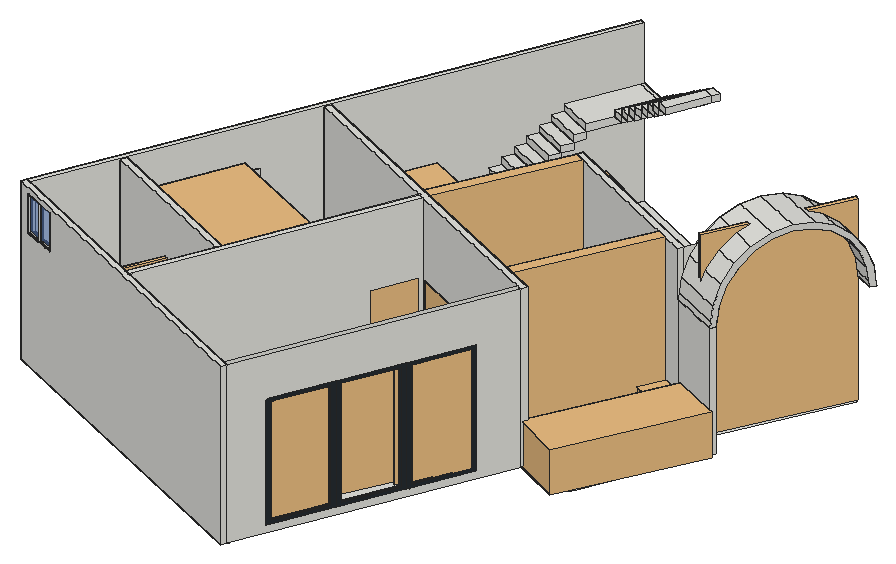
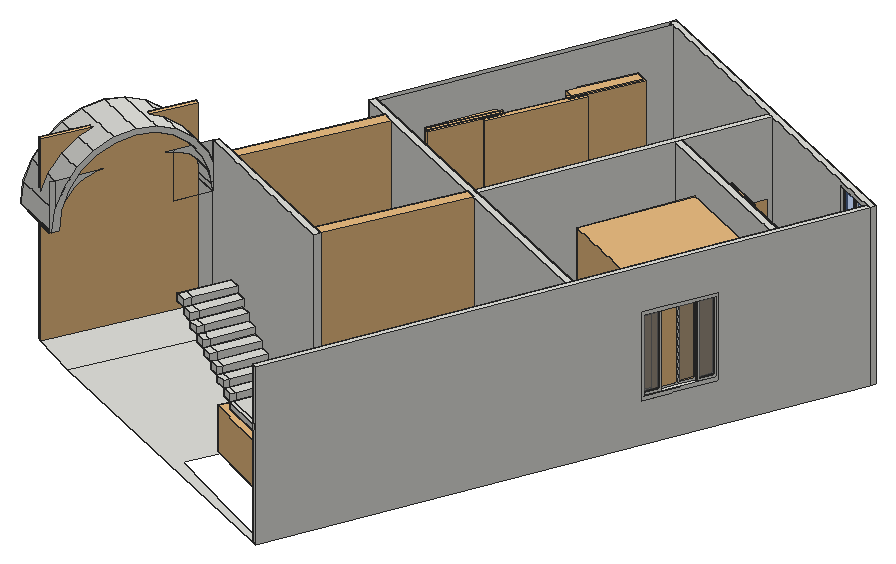
# SketchUp Ruby script. Lengths in inches.
U = 1.inch
M = Sketchup.active_model
def pt(a) = Geom::Point3d.new(a.map { |v| v * U })
def face(e, loops, mat)
  f = e.add_face(loops[0].map { |a| pt(a) })
  loops[1..].each { |l| e.add_face(l.map { |a| pt(a) }).erase! }
  f.material = f.back_material = mat if mat
  f
end
# faces: each face lists its corners as indices into pts; further lists are holes
def faces(e, pts, list, mat = nil) = list.each { |f| face(e, (f[0].is_a?(Array) ? f : [f]).map { |l| l.map { |i| pts[i] } }, mat) }
# xy, xz, yz: faces in a plane at the given z, y or x. An outline is a flat list of corners, or four numbers for a rectangle; further outlines are holes
def ring(l) = l.size == 4 ? [[l[0], l[1]], [l[2], l[1]], [l[2], l[3]], [l[0], l[3]]] : l.each_slice(2).to_a
def flat(e, list, mat, &to3) = list.each { |f| face(e, (f[0].is_a?(Array) ? f : [f]).map { |l| ring(l).map { |u, v| to3.(u, v) } }, mat) }
def xy(e, z, list, mat = nil) = flat(e, list, mat) { |x, y| [x, y, z] }
def xz(e, y, list, mat = nil) = flat(e, list, mat) { |x, z| [x, y, z] }
def yz(e, x, list, mat = nil) = flat(e, list, mat) { |y, z| [x, y, z] }
def lines(e, pts, list) = list.each { |a, b| e.add_line(pt(pts[a]), pt(pts[b])) }
# prism: a flat outline (further loops are holes) pulled along v
def prism(e, loops, v, mat = nil)
  f = face(e, loops, mat); d = Geom::Vector3d.new(v.map { |x| x * U })
  f.pushpull(f.normal.samedirection?(d) ? d.length : -d.length)
end
def box(e, o, s, mat = nil) = prism(e, [[o, [o[0] + s[0], o[1], o[2]], [o[0] + s[0], o[1] + s[1], o[2]], [o[0], o[1] + s[1], o[2]]]], [0, 0, s[2]], mat)
def at(x, y, z, deg = 0) = Geom::Transformation.translation(pt([x, y, z])) * Geom::Transformation.rotation(ORIGIN, Z_AXIS, deg.degrees)
def axes(o, x, y, z) = Geom::Transformation.new([*x, 0, *y, 0, *z, 0, *pt(o).to_a, 1])
def part(name) = M.definitions.add(name)
# library, detail: a bought-in or finely detailed component or shape, given as its bounding box
def library(name, o, s) = part(name).tap { |d| box(d.entities, o, s) }
def detail(e, o, s) = box(e.add_group.entities, o, s)
def put(e, d, t, mat = nil) = e.add_instance(d, t).tap { |i| i.material = mat if mat }
def group(e, t, mat = nil) = e.add_group.tap { |g| g.transformation = t; g.material = mat if mat }.entities
root = M.entities
M.materials.add("Wine2").color = [0, 0, 0]
M.materials["Wine2"].alpha = 0
M.materials.add("[0130_Gainsboro]").color = [39, 45, 50]
M.materials.add("[Translucent Glass Blue]").color = [100, 149, 237]
M.materials["[Translucent Glass Blue]"].alpha = 0.5
M.materials.add("[Translucent_Glass_Gray]4").color = [128, 128, 128]
M.materials["[Translucent_Glass_Gray]4"].alpha = 0.5
c1 = library("KOŁO+DRZWI+WNĘKOWE+SKRZYDŁOWE+NEXT+80,+PRAWOSTRONNE+HDRF80R\#",[0.43,0.44,0],[31.07,2.7,98.875])
c2 = library("porta 4",[0.2,-5.42,1.33],[46.55,4.72,83.21])
c3 = library("KOŁO+DRZWI+WNĘKOWE+SKRZYDŁOWE+NEXT+80,+PRAWOSTRONNE+HDRF80R",[-3.72,0,0],[35.22,3.14,98.875])
c4 = library("Group\#121",[0,0,0],[95.11,121,36.98])
c5 = library("Group\#46",[0,0,0],[59.88,84.57,74.8])
c6 = part("Group\#12")
box(c6.entities,[0,0,0],[5,144,144])
c7 = library("Bedroom furniture set",[0,-4.61,0],[113.04,95.21,114.59])
c8 = library("Group\#66",[0,0,0],[120.1,9.95,144])
c9 = library("Group\#8",[0,0,0],[126.47,47.76,36.98])
c10 = part("Group\#4")
prism(c10.entities,[[[0,298,0],[0,-5,0],[0,-5,144],[0,298,144]],[[0,39.33,108],[0,39.33,139.52],[0,7,139.52],[0,7,108]]],[5,0,0])
c11 = part("Group\#11")
prism(c11.entities,[[[0,149,0],[0,41.99,0],[0,41.99,78],[0,2.99,78],[0,2.99,0],[0,-149,0],[0,-149,144],[0,149,144]]],[5,0,0])
c12 = library("Kohler_Balast_1935.skp\#1",[-38.83,-18.45,0],[74.81,42.21,2.86])
c13 = library("window 1",[0,0,0],[3.9375,118.11,177.17])
c14 = part("Group\#74")
xy(c14.entities,0,[[0,-0.98,43.07,0],[0,0,43.07,1.4]],"[0130_Gainsboro]")
xy(c14.entities,0.3,[[0.3,-1.43,42.77,-0.98]],"[0130_Gainsboro]")
xy(c14.entities,2.95,[[2.95,-1.43,40.12,-0.63],[2.95,-0.63,40.12,0],[2.95,0,40.12,0.64],[2.95,0.64,40.12,1.4]],"[0130_Gainsboro]")
xy(c14.entities,3.54,[[3.54,-0.63,39.53,0],[3.54,0,39.53,0.64]],"[0130_Gainsboro]")
xy(c14.entities,111.8125,[[3.54,-0.63,39.53,0],[3.54,0,39.53,0.64]],"[0130_Gainsboro]")
xy(c14.entities,112.4,[[2.95,-1.43,40.12,-0.63],[2.95,-0.63,40.12,0],[2.95,0,40.12,0.64],[2.95,0.64,40.12,1.4]],"[0130_Gainsboro]")
xy(c14.entities,115.05,[[0.3,-1.43,42.77,-0.98]],"[0130_Gainsboro]")
xy(c14.entities,115.35,[[0,-0.98,43.07,0],[0,0,43.07,1.4]],"[0130_Gainsboro]")
xz(c14.entities,-1.43,[[[0.3,0.3,42.77,115.05],[2.95,2.95,40.12,112.4]]],"[0130_Gainsboro]")
xz(c14.entities,-0.98,[[[0,0,43.07,115.35],[0.3,0.3,42.77,115.05]]],"[0130_Gainsboro]")
xz(c14.entities,-0.63,[[[2.95,2.95,40.12,112.4],[3.54,3.54,39.53,111.8125]]],"[0130_Gainsboro]")
xz(c14.entities,0,[[3.54,3.54,39.53,111.8125]],"Wine2")
xz(c14.entities,0,[[[0,0,43.07,115.35],[2.95,2.95,40.12,112.4]],[[2.95,2.95,40.12,112.4],[3.54,3.54,39.53,111.8125]]],"[0130_Gainsboro]")
xz(c14.entities,0.64,[[[2.95,2.95,40.12,112.4],[3.54,3.54,39.53,111.8125]]],"[0130_Gainsboro]")
xz(c14.entities,1.4,[[[0,0,43.07,115.35],[2.95,2.95,40.12,112.4]]],"[0130_Gainsboro]")
yz(c14.entities,0,[[-0.98,0,0,115.35],[0,0,1.4,115.35]],"[0130_Gainsboro]")
yz(c14.entities,0.3,[[-1.43,0.3,-0.98,115.05]],"[0130_Gainsboro]")
yz(c14.entities,2.95,[[-1.43,2.95,-0.63,112.4],[-0.63,2.95,0,112.4],[0,2.95,0.64,112.4],[0.64,2.95,1.4,112.4]],"[0130_Gainsboro]")
yz(c14.entities,3.54,[[-0.63,3.54,0,111.8125],[0,3.54,0.64,111.8125]],"[0130_Gainsboro]")
yz(c14.entities,39.53,[[-0.63,3.54,0,111.8125],[0,3.54,0.64,111.8125]],"[0130_Gainsboro]")
yz(c14.entities,40.12,[[-1.43,2.95,-0.63,112.4],[-0.63,2.95,0,112.4],[0,2.95,0.64,112.4],[0.64,2.95,1.4,112.4]],"[0130_Gainsboro]")
yz(c14.entities,42.77,[[-1.43,0.3,-0.98,115.05]],"[0130_Gainsboro]")
yz(c14.entities,43.07,[[-0.98,0,0,115.35],[0,0,1.4,115.35]],"[0130_Gainsboro]")
c15 = part("Glazed door assembly")
put(c15.entities,c14,axes([90.57,1.43,0],[1.05148,0,0],[0,1,0],[0,0,1]))
put(c15.entities,c14,axes([0,1.43,0],[1.05148,0,0],[0,1,0],[0,0,1]))
put(c15.entities,c14,axes([45.29,1.43,0],[1.05148,0,0],[0,1,0],[0,0,1]))
c16 = library("Group8\#1",[-48.75,-20.06,-0.03],[97.5,40.12,31.8])
c17 = library("3d flower - flower pot",[-12.2,-15.73,0],[29.88,29.15,27.8])
c18 = library("Dining table set",[0,0,0],[65.45,109.33,43.4])
c19 = library("Group14",[-64.97,9.24,0.31],[138.52,9.93,292.57])
c20 = library("Group16",[86.37,-10.76,76.46],[21.79,14.87,35.97])
c21 = library("Group22",[48.82,-10.91,0.23],[97.72,18.57,293.12])
c22 = library("Group24",[44.03,2.01,0.26],[103.73,11,292.35])
c23 = library("Group27",[-106.21,-10.76,76.46],[21.8,14.87,35.97])
c24 = library("Group35",[-145.81,2.01,0.26],[103.73,11,292.35])
c25 = library("Group33",[-144.59,-10.91,0.23],[97.72,18.57,293.12])
c26 = part("Group\#71")
put(c26.entities,c19,at(145.81,10.91,-0.23))
put(c26.entities,c20,at(145.81,10.91,-0.23))
put(c26.entities,c21,at(145.81,10.91,-0.23))
put(c26.entities,c22,at(145.81,10.91,-0.23))
put(c26.entities,c23,at(145.81,10.91,-0.23))
put(c26.entities,c24,at(145.81,10.91,-0.23))
put(c26.entities,c25,at(145.81,10.91,-0.23))
c27 = library("Group13\#1",[-103.57,-19.82,-0.03],[42.43,40.67,31.4])
c28 = part("Group\#117")
xy(c28.entities,0,[[0,0,36,10]])
g1 = group(c28.entities,at(-0.41,0,0))
g2 = group(g1,at(0,0,0))
xy(g2,6,[[0.41,0,36.41,10]])
xz(g2,0,[[0.41,0,36.41,6]])
xz(g2,10,[[0.41,0,36.41,6]])
yz(g2,0.41,[[0,0,10,6]])
yz(g2,36.41,[[0,0,10,6]])
c29 = library("bathroom kit",[-10.19,-11.89,-0.14],[22.08,39.51,30.77])
c30 = library("Shower_03.skp",[-9.2,-8.46,-0.03],[13.92,58.47,24.25])
c31 = part("Component\#36")
prism(c31.entities,[[[0,70.87,0],[0,0,0],[0,0,47.24],[0,70.87,47.24]],[[0,1.97,1.97],[0,68.9,1.97],[0,68.9,45.28],[0,1.97,45.28]]],[7.875,0,0])
c32 = part("Component\#34")
xy(c32.entities,0,[[0,0,3.9375,16.73]])
xy(c32.entities,0.98,[[0,0.98,1.77,15.75],[1.77,0.98,2.85,15.75],[2.85,0.98,3.9375,15.75]])
xy(c32.entities,42.32,[[0,0.98,1.77,15.75],[1.77,0.98,2.85,15.75],[2.85,0.98,3.9375,15.75]])
xy(c32.entities,43.31,[[0,0,3.9375,16.73]])
xz(c32.entities,0,[[0,0,3.9375,43.31]])
xz(c32.entities,0.98,[[0,0.98,1.77,42.32],[1.77,0.98,2.85,42.32],[2.85,0.98,3.9375,42.32]])
xz(c32.entities,15.75,[[0,0.98,1.77,42.32],[1.77,0.98,2.85,42.32],[2.85,0.98,3.9375,42.32]])
xz(c32.entities,16.73,[[0,0,3.9375,43.31]])
yz(c32.entities,0,[[[0,0,16.73,43.31],[0.98,0.98,15.75,42.32]]])
yz(c32.entities,1.77,[[0.98,0.98,15.75,42.32]],"[Translucent_Glass_Gray]4")
yz(c32.entities,2.85,[[0.98,0.98,15.75,42.32]],"[Translucent_Glass_Gray]4")
yz(c32.entities,3.9375,[[[0,0,16.73,43.31],[0.98,0.98,15.75,42.32]]])
c33 = part("simple window")
p = [[0,68.9,1.97],[0,35.43,1.97]]
lines(c33.entities,p,[[0,1]])
put(c33.entities,c31,at(0,0,0))
put(c33.entities,c32,axes([1.14,52.17,1.97],[0.71,0,0],[0,1,0],[0,0,1]))
put(c33.entities,c32,axes([1.14,1.97,1.97],[0.71,0,0],[0,1,0],[0,0,1]))
put(c33.entities,c32,axes([3.9375,18.7,1.97],[0.71,0,0],[0,1,0],[0,0,1]))
put(c33.entities,c32,axes([3.9375,35.43,1.97],[0.71,0,0],[0,1,0],[0,0,1]))
c34 = part("Group\#67")
xy(c34.entities,0,[[0,0,36,10]])
g3 = group(c34.entities,at(-0.41,0,0))
g4 = group(g3,at(0,0,0))
xy(g4,6,[[0.41,0,36.41,35.24]])
xz(g4,0,[[0.41,0,36.41,6]])
xz(g4,35.24,[[0.41,0,36.41,6]])
yz(g4,0.41,[[0,0,35.24,6]])
yz(g4,36.41,[[0,0,35.24,6]])
c35 = part("Group\#53")
xy(c35.entities,0,[[0,0,36,10]])
g5 = group(c35.entities,at(-0.41,0,0))
g6 = group(g5,at(0,0,0))
xy(g6,6,[[0.41,0,36.41,10]])
xz(g6,0,[[0.41,0,36.41,6]])
xz(g6,10,[[0.41,0,36.41,6]])
yz(g6,0.41,[[0,0,10,6]])
yz(g6,36.41,[[0,0,10,6]])
c36 = part("Janela aluminio")
xy(c36.entities,0,[[0,0,47.24,1.57],[23.62,1.57,47.24,2.76],[0,2.76,25.98,3.9375],[0,3.9375,47.24,5.91]])
xy(c36.entities,43.31,[[0,0,47.24,1.57],[23.62,1.57,47.24,2.76],[0,2.76,0,5.91,47.24,5.91,47.24,3.9375,25.98,3.9375,25.98,2.76],[25.98,2.76,47.24,3.9375]])
xz(c36.entities,1.57,[[0,0,23.62,0,23.62,41.34,21.26,41.34,21.26,1.97,1.97,1.97,1.97,41.34,23.62,41.34,23.62,43.31,0,43.31],[[23.62,0,47.24,43.31],[25.7,1.97,45.28,41.34]]])
xz(c36.entities,2.76,[[[0,0,23.62,43.31],[2.36,2.36,21.26,40.94]],[23.62,0,25.98,43.31]])
xz(c36.entities,2.76,[[2.36,2.36,21.26,40.94]],"[Translucent Glass Blue]")
xz(c36.entities,3.9375,[[25.98,0,25.98,2.36,44.88,2.36,44.88,40.94,25.98,40.94,25.98,43.31,47.24,43.31,47.24,0]])
xz(c36.entities,3.9375,[[25.98,2.36,44.88,40.94]],"[Translucent Glass Blue]")
yz(c36.entities,0,[[0,0,1.57,43.31],[2.76,0,5.91,43.31]])
yz(c36.entities,23.62,[[1.57,0,2.76,43.31]])
yz(c36.entities,25.98,[[2.76,0,3.9375,43.31]])
yz(c36.entities,47.24,[[0,0,1.57,43.31],[1.57,0,2.76,43.31],[3.9375,0,5.91,43.31]])
xy(root,162,[[[839.724,541.426,841.717,546.01,837.135,548.006,930.972,763.458,935.556,761.462,957.103,750.999,959.962,749.841,960.919,749.596,962.951,749.076,964.937,748.845,966.015,748.719,969.099,748.775,972.148,749.245,975.106,750.118,977.921,751.38,980.541,753.008,982.92,754.972,985.014,757.237,986.785,759.762,988.203,762.502,1021.036,838.006,1021.052,838.042,1022.099,840.815,1022.739,843.75,1022.942,846.747,1022.704,849.741,1022.032,852.669,1020.938,855.466,1019.447,858.074,1017.591,860.436,1015.41,862.5,1013.436,863.883,1007.411,866.508,1010.264,865.569,1012.95,864.224,1013.436,863.883,1029.287,856.98,1031.281,861.565,1031.219,861.592,1028.364,862.835,1027.135,860.303,1008.199,869.498,965.832,890.07,1020.479,1002.61,764.166,1114.243,759.581,1116.239,561.938,662.44],[754.403,984.89,718.473,1002.337,769.05,1106.497,805.201,1089.503,874.577,1055.816,861.065,1027.987,791.688,1061.675]],[841.72,546.009,934.755,759.624,934.632,759.678,841.717,546.01],[841.717,546.01,934.632,759.678,934.755,759.624,935.556,761.462,930.972,763.458,837.135,548.006],[1021.038,838.005,1021.052,838.042,1021.036,838.006],[1029.476,856.897,1031.472,861.482,1031.283,861.564,1029.289,856.979],
  [1029.289,856.979,1031.283,861.564,1031.281,861.565,1029.287,856.98],[1027.135,860.303,1028.364,862.835,1009.049,871.248,1008.777,870.687,1008.56,870.241,1008.321,869.75,1008.199,869.498],[1013.436,863.883,1012.95,864.224,1010.264,865.569,1007.411,866.508],[1008.199,869.498,1008.321,869.75,972.0625,887.356,965.832,890.07],[1008.321,869.75,1008.56,870.241,984.197,882.071,972.0625,887.356],
  [1008.56,870.241,1008.777,870.687,995.208,877.276,984.197,882.071],[1008.777,870.687,1009.049,871.248,995.208,877.276],[1009.049,871.248,1062.846,982.038,1020.479,1002.61,965.832,890.07,972.0625,887.356,984.197,882.071,995.208,877.276]])
xy(root,168,[[854.098,574.43,921.181,728.456,916.597,730.453,849.514,576.427]])
xy(root,264.897,[[1080.487,974.318,1082.673,978.819,1039.564,999.752,1037.378,995.251]])
xy(root,270,[[854.098,574.43,849.514,576.427,916.597,730.453,921.181,728.456]])
p = [[837.135,548.006,162],[841.717,546.01,162],[841.72,546.009,162],[841.72,546.009,306],[837.135,548.006,306],[934.755,759.624,162],
  [935.556,761.462,162],[935.556,761.462,306],[854.098,574.43,168],[854.098,574.43,270],[921.181,728.456,270],[921.181,728.456,168],
  [930.972,763.458,306],[930.972,763.458,162],[916.597,730.453,168],[916.597,730.453,270],[849.514,576.427,270],[849.514,576.427,168],
  [999.843,909.07,306],[987.465,880.648,306],[987.465,880.648,300.738],[987.465,880.648,264.897],[987.59,880.934,269.962],[987.961,881.788,274.952],
  [988.575,883.196,279.789],[989.421,885.138,284.402],[990.486,887.585,288.719],[991.755,890.498,292.677],[993.208,893.835,296.215],[994.824,897.544,299.279],
  [996.577,901.57,301.824],[998.442,905.852,303.811],[999.843,909.069,304.818],[1037.253,994.964,269.962],[1037.378,995.251,264.897],[1037.378,995.251,306],
  [1022.45,960.977,306],[1024.452,965.573,305.21],[1026.401,970.046,303.811],[1028.266,974.328,301.824],[1030.019,978.355,299.279],[1031.635,982.064,296.215],
  [1033.088,985.401,292.677],[1034.357,988.314,288.719],[1035.422,990.76,284.402],[1036.268,992.702,279.789],[1036.881,994.111,274.952],[1039.564,999.752,306],
  [1039.564,999.752,264.897],[1000.39,910.325,305.21],[1002.392,914.922,306],[1031.219,861.592,168],[1031.472,861.482,168],[987.465,880.648,168],
  [985.468,876.064,168],[1031.219,861.592,162],[963.643,885.561,162],[965.832,890.07,162],[764.166,1114.243,162],[750.288,1085.662,162],
  [999.843,909.069,264.897]]
faces(root,p,[[0,1,2,3,4],[[3,2,5,6,7],[8,9,10,11]],[[12,13,0,4],[14,15,16,17]],[6,13,12,7],[8,17,16,9],[10,15,14,11],[18,19,20,21,22,23,24,25,26,27,28,29,30,31,32],[33,34,35,36,37,38,39,40,41,42,43,44,45,46],
  [47,35,34,48],[32,49,50,18]])
lines(root,p,[[51,52],[53,54],[51,55],[56,57],[58,59],[21,60],[60,32]])
put(root,c1,axes([680.21,652.39,161.99],[-1.10532,0.49586,0],[0.40931,0.9124,0],[0,0,1]))
put(root,c1,axes([681.01,655.04,161.99],[1.10532,-0.49586,0],[-0.40931,-0.9124,0],[0,0,1]))
put(root,c2,axes([837.12,803.24,160.74],[-0.76347,0.34639,0],[-0.41316,-0.91066,0],[0,0,0.93759]))
put(root,c3,axes([646.6,668.76,162],[0.48304,1.08503,0],[-0.91356,0.4067,0],[0,0,1]))
put(root,c4,at(823.78,942.11,162,64.1))
put(root,c5,at(664.81,885.02,162,-23.435))
put(root,c6,at(599.32,735.6,162,-113.535))
put(root,c7,at(601.37,738.72,162,-23.1))
g7 = group(root,at(846.27,942.14,162,-113.535))
xy(g7,0,[[0,0,5,202]])
xy(g7,102.9,[[0,154,5,202]])
xy(g7,144,[[0,0,5,154]])
xz(g7,0,[[0,0,5,144]])
xz(g7,154,[[0,102.9,5,144]])
xz(g7,202,[[0,0,5,102.9]])
yz(g7,0,[[0,0,154,144],[154,0,202,102.9]])
yz(g7,5,[[0,0,154,144],[154,0,202,102.9]])
p = [[1.32,162.39,0],[0,162.45,0]]
lines(g7,p,[[0,1]])
g8 = group(root,at(717.26,1019.06,162,-113.535))
prism(g8,[[[-106,0,0],[384,0,0],[384,0,144],[-106,0,144]],[[203.27,0,108],[263.27,0,108],[263.27,0,36],[203.27,0,36]]],[0,5,0])
g9 = group(root,at(705.02,605.32,162,64.1))
xy(g9,0,[[0.21,0,0,5,3.03,5.12,3.23,0.125],[42.2,1.73,41.99,6.73,192.84,12.96,193.04,7.97],[193.04,7.97,232.01,9.58,231.8,14.57,192.84,12.96],[232.01,9.58,231.8,14.57,234.8,14.69,235.01,9.7]])
xy(g9,78,[[3.23,0.125,3.03,5.12,41.99,6.73,42.2,1.73]])
xy(g9,79.24,[[193.04,7.97,192.84,12.96,231.8,14.57,232.01,9.58]])
xy(g9,144,[[0.21,0,3.23,0.125,235.01,9.7,234.8,14.69,0,5]])
p = [[0,5,0],[0.21,0,0],[0.21,0,144],[0,5,144],[3.23,0.125,0],[3.23,0.125,78],
  [3.23,0.125,144],[3.03,5.12,0],[3.03,5.12,78],[235.01,9.7,144],[42.2,1.73,78],[42.2,1.73,0],
  [193.04,7.97,0],[193.04,7.97,79.24],[232.01,9.58,79.24],[232.01,9.58,0],[235.01,9.7,0],[41.99,6.73,78],
  [41.99,6.73,0],[234.8,14.69,0],[231.8,14.57,0],[231.8,14.57,79.24],[192.84,12.96,79.24],[192.84,12.96,0],
  [234.8,14.69,144]]
faces(g9,p,[[0,1,2,3],[4,5,6,2,1],[5,4,7,8],[9,6,5,10,11,12,13,14,15,16],[11,10,17,18],[19,20,21,22,23,18,17,8,7,0,3,24],[13,12,23,22],[15,14,21,20],
  [16,19,24,9]])
put(root,c8,at(959.15,887.74,162,-115.9))
put(root,c9,at(977.0625,742.33,162,64.1))
put(root,c10,at(568.52,665.03,162,-113.535))
put(root,c11,at(800.95,825.54,162,-113.535))
put(root,c8,at(844.55,937.65,162,-115.9))
put(root,c12,axes([687.53,674.23,162],[-0.91179,0.41065,0],[-0.36093,-0.80138,0],[0,0,1]))
put(root,c2,axes([722.34,644.03,160.76],[-0.33455,-0.76814,0],[0.91682,-0.3993,0],[0,0,0.93749]))
put(root,c2,axes([798.2,818.2,162],[-0.33455,-0.76814,0],[0.91682,-0.3993,0],[0,0,0.93749]))
put(root,c13,axes([1063.15,982.66,164],[-0.89956,0.4368,0],[-0.4538,-0.93456,0],[0,0,0.91978]))
put(root,c15,axes([854.07,574.36,167.73],[0.49513,1.13686,0],[-0.91682,0.3993,0],[0,0,0.89]))
put(root,c16,axes([922.57,854,168.02],[-0.37135,-0.85264,0],[0.91682,-0.3993,0],[0,0,0.79]))
put(root,c17,axes([968.74,869.03,168],[0.35381,0.72864,0],[-0.72864,0.35381,0],[0,0,0.81]))
put(root,c18,axes([901.1875,706.89,168],[0.34729,0.84112,0],[-0.84112,0.34729,0],[0,0,0.91]))
put(root,c26,axes([846.74,575.16,168],[0.25356,0.52218,0],[-0.45877,0.22277,0],[0,0,0.3672]))
put(root,c27,at(892.48,973.34,168.03,64.1))
put(root,c28,at(795.4,925.84,168,66.285))
put(root,c29,at(618.6,710.1,169.64,-115.9))
put(root,c28,at(786.25,929.86,174,66.285))
put(root,c28,at(777.09,933.88,180,66.285))
put(root,c28,at(767.9375,937.9,186,66.285))
put(root,c28,at(758.78,941.93,192,66.285))
put(root,c30,axes([721.72,656.52,201.85],[-0.37601,-0.92662,0],[0,0,1],[-0.92662,0.37601,0]))
put(root,c33,axes([612.13,777.68,198],[0.91682,-0.3993,0],[0.34739,0.79763,0],[0,0,1.524]))
put(root,c28,at(749.625,945.95,198,66.285))
put(root,c28,at(740.47,949.97,204,66.285))
put(root,c34,at(731.3125,953.99,210,66.285))
put(root,c28,at(749.8125,996.11,216,156.285))
put(root,c28,at(753.84,1005.26,222,156.285))
put(root,c28,at(757.86,1014.42,228,156.285))
put(root,c28,at(761.88,1023.57,234,156.285))
put(root,c28,at(765.9,1032.73,240,156.285))
put(root,c35,at(769.92,1041.89,246,156.285))
g10 = group(root,at(769.92,1041.89,252,66.285))
xy(g10,0,[[0,0,36,10]])
g11 = group(g10,at(-0.41,0,0))
g12 = group(g11,at(0,0,0))
xy(g12,0,[[61.41,0,64.39,35.24]])
xy(g12,6,[[0.41,0,61.41,35.24],[61.41,0,64.39,35.24]])
xz(g12,0,[[0.41,0,61.41,6],[61.41,0,64.39,6]])
xz(g12,35.24,[[0.41,0,61.41,6],[61.41,0,64.39,6]])
yz(g12,0.41,[[0,0,35.24,6]])
yz(g12,64.39,[[0,0,35.24,6]])
g13 = group(root,at(788.375,1059.03,258,66.285))
xy(g13,0,[[0,0,36,10]])
g14 = group(g13,at(-0.41,0,0))
g15 = group(g14,at(0,0,0))
xy(g15,0,[[36.41,0,41.28,10]])
xy(g15,6,[[0.41,0,36.41,10],[36.41,0,41.28,10]])
xz(g15,0,[[0.41,0,36.41,6],[36.41,0,41.28,6]])
xz(g15,10,[[0.41,0,36.41,6],[36.41,0,41.28,6]])
yz(g15,0.41,[[0,0,10,6]])
yz(g15,41.28,[[0,0,10,6]])
g16 = group(root,at(797.53,1055,264,66.285))
xy(g16,0,[[0,0,36,10]])
g17 = group(g16,at(-0.41,0,0))
g18 = group(g17,at(0,0,0))
xy(g18,0,[[36.41,0,41.36,10]])
xy(g18,6,[[0.41,0,36.41,10],[36.41,0,41.36,10]])
xz(g18,0,[[0.41,0,36.41,6],[36.41,0,41.36,6]])
xz(g18,10,[[0.41,0,36.41,6],[36.41,0,41.36,6]])
yz(g18,0.41,[[0,0,10,6]])
yz(g18,41.36,[[0,0,10,6]])
g19 = group(root,at(1028.46,854.82,264.9))
xy(g19,0.01,[[52.03,119.51,9.22,138.11,11.22,142.73,54.04,124.13]])
p = [[12.15,144.85,-0.32],[9.93,140.37,-0.32],[51.82,119.64,0.01],[54.04,124.13,0.01],[3.02,6.7,0],[1.02,2.07,0],
  [-41.8,20.68,0.01],[-39.79,25.3,0.01],[3.29,7.3,5],[-39.53,25.9,5],[52.03,119.51,0.01],[51.77,118.9,5],
  [8.96,137.5,5.01],[9.22,138.11,0.01],[1.33,2.71,0],[3.05,6.64,0]]
faces(g19,p,[[0,1,2,3],[4,5,6,7],[8,4,7,9],[10,11,12,13]])
lines(g19,p,[[14,15],[8,15],[5,14]])
g20 = group(g19,at(0,0,0))
p = [[1.02,2.07,0],[1.3,2.72,5.36],[-42.82,21.89,5.37],[-43.1,21.24,0.01],[3.02,6.7,0],[3.29,7.3,5],
  [3.86,8.62,15.92],[6.31,14.25,30.75],[10.2,23.21,43.49],[15.28,34.89,53.26],[21.19,48.5,59.41],[27.53,63.1,61.5],
  [33.875,77.69,59.41],[39.78,91.3,53.27],[44.86,102.98,43.49],[48.75,111.95,30.76],[51.2,117.58,15.93],[51.77,118.9,5],
  [52.03,119.51,0.01],[54.04,124.13,0.01],[53.14,122.05,17.23],[50.49,115.95,33.28],[46.28,106.25,47.06],[40.79,93.61,57.63],
  [34.4,78.89,64.28],[27.53,63.1,66.54],[20.67,47.3,64.27],[14.28,32.58,57.625],[8.78,19.94,47.05],[4.57,10.25,33.27],
  [1.92,4.15,17.22],[-40.83,26.46,5],[-41.09,25.86,0.01],[-42.2,23.32,17.23],[-39.55,29.41,33.28],[-35.33,39.11,47.06],
  [-29.84,51.75,57.63],[-23.44,66.47,64.28],[-16.58,82.26,66.55],[-9.72,98.06,64.28],[-3.33,112.78,57.64],[2.16,125.42,47.0625],
  [6.375,135.12,33.28],[9.02,141.21,17.24],[9.92,143.29,0.01],[7.92,138.67,0.01],[7.66,138.07,5.01],[7.08,136.75,15.93],
  [4.64,131.11,30.76],[0.74,122.15,43.5],[-4.33,110.47,53.27],[-10.24,96.86,59.41],[-16.58,82.26,61.51],[-22.93,67.66,59.41],
  [-28.84,54.06,53.27],[-33.91,42.38,43.49],[-37.81,33.42,30.76],[-40.26,27.78,15.92]]
faces(g20,p,[[0,1,2,3],[4,5,6,7,8,9,10,11,12,13,14,15,16,17,18,19,20,21,22,23,24,25,26,27,28,29,30,1,0],[31,32,3,2,33,34,35,36,37,38,39,40,41,42,43,44,45,46,47,48,49,50,51,52,53,54,55,56,57],[20,19,44,43],[6,5,31,57],[17,16,47,46],[1,30,33,2],[7,6,57,56],
  [16,15,48,47],[30,29,34,33],[21,20,43,42],[8,7,56,55],[15,14,49,48],[29,28,35,34],[22,21,42,41],[9,8,55,54],
  [14,13,50,49],[28,27,36,35],[23,22,41,40],[10,9,54,53],[13,12,51,50],[27,26,37,36],[24,23,40,39],[11,10,53,52],
  [12,11,52,51],[26,25,38,37],[25,24,39,38]])
g21 = group(root,at(806.6875,1050.98,270,66.285))
xy(g21,0,[[0,0,36,10]])
g22 = group(g21,at(-0.41,0,0))
g23 = group(g22,at(0,0,0))
xy(g23,0,[[36.41,0,41.36,10]])
xy(g23,6,[[0.41,0,36.41,10],[36.41,0,41.36,10]])
xz(g23,0,[[0.41,0,36.41,6],[36.41,0,41.36,6]])
xz(g23,10,[[0.41,0,36.41,6],[36.41,0,41.36,6]])
yz(g23,0.41,[[0,0,10,6]])
yz(g23,41.36,[[0,0,10,6]])
put(root,c36,axes([603.66,647.27,270.32],[-0.62484,0.2578,0],[-0.1373,-0.33279,0],[0,0,0.72049]))
g24 = group(root,at(815.84,1046.96,276,66.285))
xy(g24,0,[[0,0,36,10]])
g25 = group(g24,at(-0.41,0,0))
g26 = group(g25,at(0,0,0))
xy(g26,0,[[36.41,0,41.39,10]])
xy(g26,6,[[0.41,0,36.41,10],[36.41,0,41.39,10]])
xz(g26,0,[[0.41,0,36.41,6],[36.41,0,41.39,6]])
xz(g26,10,[[0.41,0,36.41,6],[36.41,0,41.39,6]])
yz(g26,0.41,[[0,0,10,6]])
yz(g26,41.39,[[0,0,10,6]])
g27 = group(root,at(825,1042.9375,282,66.285))
xy(g27,0,[[0,0,36,10]])
g28 = group(g27,at(-0.41,0,0))
g29 = group(g28,at(0,0,0))
xy(g29,0,[[36.41,0,41.8,10]])
xy(g29,6,[[0.41,0,36.41,10],[36.41,0,41.8,10]])
xz(g29,0,[[0.41,0,36.41,6],[36.41,0,41.8,6]])
xz(g29,10,[[0.41,0,36.41,6],[36.41,0,41.8,6]])
yz(g29,0.41,[[0,0,10,6]])
yz(g29,41.8,[[0,0,10,6]])
g30 = group(root,at(834.15,1038.92,288,66.285))
xy(g30,0,[[0,0,36,10]])
g31 = group(g30,at(-0.41,0,0))
g32 = group(g31,at(0,0,0))
xy(g32,0,[[36.41,0,41.8,10]])
xy(g32,6,[[0.41,0,36.41,10],[36.41,0,41.8,10]])
xz(g32,0,[[0.41,0,36.41,6],[36.41,0,41.8,6]])
xz(g32,10,[[0.41,0,36.41,6],[36.41,0,41.8,6]])
yz(g32,0.41,[[0,0,10,6]])
yz(g32,41.8,[[0,0,10,6]])
g33 = group(root,at(842.75,1033.3125,294,66.285))
xy(g33,0,[[0,0,36,10]])
g34 = group(g33,at(-0.41,0,0))
g35 = group(g34,at(0,0,0))
xy(g35,0,[[36.41,0,43.47,10]])
xy(g35,6,[[0.41,0,36.41,10],[36.41,0,43.47,10]])
xz(g35,0,[[0.41,0,36.41,6],[36.41,0,43.47,6]])
xz(g35,10,[[0.41,0,36.41,6],[36.41,0,43.47,6]])
yz(g35,0.41,[[0,0,10,6]])
yz(g35,43.47,[[0,0,10,6]])
g36 = group(root,at(851.91,1029.29,300,66.285))
xy(g36,0,[[0,0,36,10]])
g37 = group(g36,at(-0.41,0,0))
g38 = group(g37,at(0,0,0))
xy(g38,0,[[36.41,0,43.49,10]])
xy(g38,6,[[0.41,0,36.41,10],[36.41,0,43.49,10]])
xz(g38,0,[[0.41,0,36.41,6],[36.41,0,43.49,6]])
xz(g38,10,[[0.41,0,36.41,6],[36.41,0,43.49,6]])
yz(g38,0.41,[[0,0,10,6]])
yz(g38,43.49,[[0,0,10,6]])
